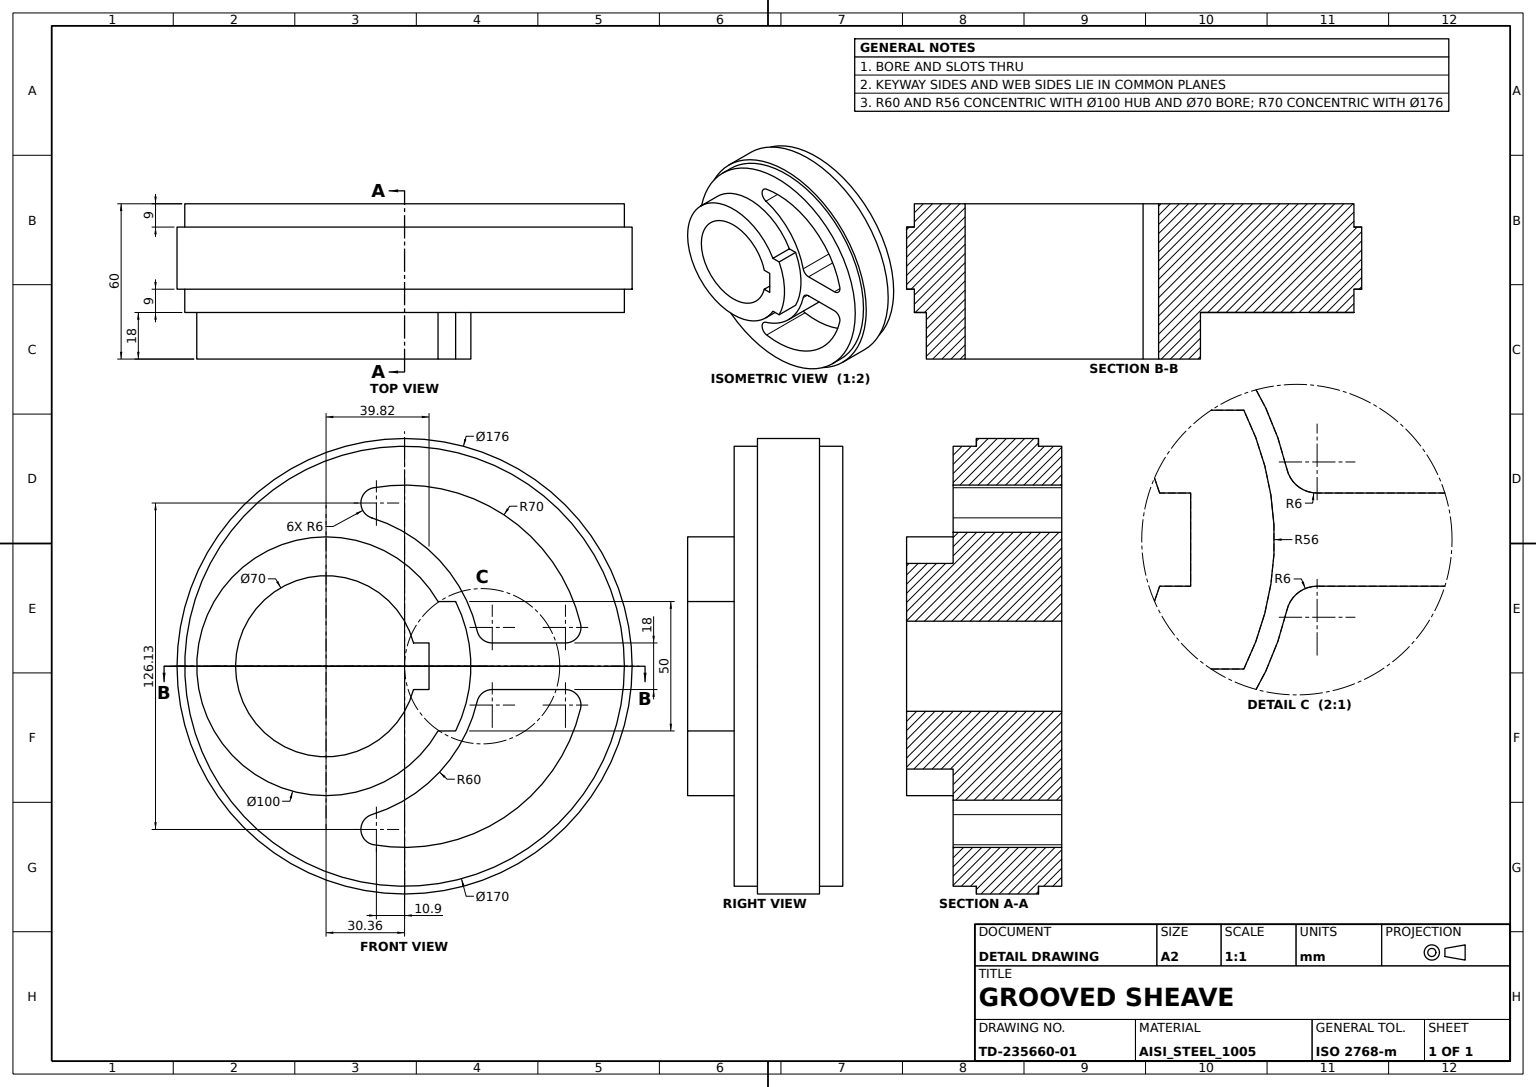
ISO-10303-21;
HEADER;
FILE_DESCRIPTION((''),'2;1');
FILE_NAME('','',(''),(''),'','','');
FILE_SCHEMA(('AUTOMOTIVE_DESIGN'));
ENDSEC;
DATA;
#1=APPLICATION_CONTEXT('');
#2=PRODUCT_CONTEXT('',#1,'mechanical');
#3=PRODUCT('','','',(#2));
#4=PRODUCT_DEFINITION_FORMATION('','',#3);
#5=PRODUCT_DEFINITION_CONTEXT('',#1,'design');
#6=PRODUCT_DEFINITION('','',#4,#5);
#7=PRODUCT_DEFINITION_SHAPE('','',#6);
#8=(LENGTH_UNIT()NAMED_UNIT(*)SI_UNIT(.MILLI.,.METRE.));
#9=(NAMED_UNIT(*)PLANE_ANGLE_UNIT()SI_UNIT($,.RADIAN.));
#10=(NAMED_UNIT(*)SI_UNIT($,.STERADIAN.)SOLID_ANGLE_UNIT());
#11=UNCERTAINTY_MEASURE_WITH_UNIT(LENGTH_MEASURE(0.005),#8,'distance_accuracy_value','');
#12=(GEOMETRIC_REPRESENTATION_CONTEXT(3)GLOBAL_UNCERTAINTY_ASSIGNED_CONTEXT((#11))GLOBAL_UNIT_ASSIGNED_CONTEXT((#8,#9,#10))REPRESENTATION_CONTEXT('',''));
#13=CARTESIAN_POINT('',(0.,85.,12.));
#14=VERTEX_POINT('',#13);
#15=CARTESIAN_POINT('',(0.,0.,12.));
#16=DIRECTION('',(0.,0.,1.));
#17=DIRECTION('',(0.,1.,0.));
#18=AXIS2_PLACEMENT_3D('',#15,#16,#17);
#19=CIRCLE('',#18,85.);
#20=EDGE_CURVE('',#14,#14,#19,.T.);
#21=ORIENTED_EDGE('',*,*,#20,.F.);
#22=EDGE_LOOP('',(#21));
#23=FACE_BOUND('',#22,.T.);
#24=CARTESIAN_POINT('',(0.,88.,12.));
#25=VERTEX_POINT('',#24);
#26=CIRCLE('',#18,88.);
#27=EDGE_CURVE('',#25,#25,#26,.T.);
#28=ORIENTED_EDGE('',*,*,#27,.T.);
#29=EDGE_LOOP('',(#28));
#30=FACE_BOUND('',#29,.T.);
#31=DIRECTION('',(1.,0.,0.));
#32=AXIS2_PLACEMENT_3D('',#15,#16,#31);
#33=PLANE('',#32);
#34=ADVANCED_FACE('',(#23,#30),#33,.T.);
#35=CARTESIAN_POINT('',(-13.636364,28.067483,-21.));
#36=VERTEX_POINT('',#35);
#37=CARTESIAN_POINT('',(-57.331854,-12.668926,-21.));
#38=VERTEX_POINT('',#37);
#39=CARTESIAN_POINT('',(0.,-30.362386,-21.));
#40=AXIS2_PLACEMENT_3D('',#39,#16,#31);
#41=CIRCLE('',#40,60.);
#42=EDGE_CURVE('',#36,#38,#41,.T.);
#43=ORIENTED_EDGE('',*,*,#42,.T.);
#44=CARTESIAN_POINT('',(-57.331854,-12.668926,21.));
#45=VERTEX_POINT('',#44);
#46=CARTESIAN_POINT('',(-57.331854,-12.668926,-54979.));
#47=VECTOR('',#16,1000.);
#48=LINE('',#46,#47);
#49=EDGE_CURVE('',#45,#38,#48,.F.);
#50=ORIENTED_EDGE('',*,*,#49,.F.);
#51=CARTESIAN_POINT('',(-13.636364,28.067483,21.));
#52=VERTEX_POINT('',#51);
#53=CARTESIAN_POINT('',(0.,-30.362386,21.));
#54=DIRECTION('',(0.,0.,-1.));
#55=AXIS2_PLACEMENT_3D('',#53,#54,#31);
#56=CIRCLE('',#55,60.);
#57=EDGE_CURVE('',#45,#52,#56,.T.);
#58=ORIENTED_EDGE('',*,*,#57,.T.);
#59=CARTESIAN_POINT('',(-13.636364,28.067483,-54979.));
#60=LINE('',#59,#47);
#61=EDGE_CURVE('',#52,#36,#60,.F.);
#62=ORIENTED_EDGE('',*,*,#61,.T.);
#63=EDGE_LOOP('',(#43,#50,#58,#62));
#64=FACE_BOUND('',#63,.T.);
#65=CARTESIAN_POINT('',(0.,-30.362386,-54979.));
#66=AXIS2_PLACEMENT_3D('',#65,#16,#31);
#67=CYLINDRICAL_SURFACE('',#66,60.);
#68=ADVANCED_FACE('',(#64),#67,.T.);
#69=CARTESIAN_POINT('',(-9.,3.460683,39.));
#70=VERTEX_POINT('',#69);
#71=CARTESIAN_POINT('',(-9.,3.460683,-21.));
#72=VERTEX_POINT('',#71);
#73=VECTOR('',#54,1000.);
#74=LINE('',#69,#73);
#75=EDGE_CURVE('',#70,#72,#74,.T.);
#76=ORIENTED_EDGE('',*,*,#75,.F.);
#77=CARTESIAN_POINT('',(9.,3.460683,39.));
#78=VERTEX_POINT('',#77);
#79=CARTESIAN_POINT('',(0.,-30.362386,39.));
#80=AXIS2_PLACEMENT_3D('',#79,#54,#31);
#81=CIRCLE('',#80,35.);
#82=EDGE_CURVE('',#78,#70,#81,.T.);
#83=ORIENTED_EDGE('',*,*,#82,.F.);
#84=CARTESIAN_POINT('',(9.,3.460683,-21.));
#85=VERTEX_POINT('',#84);
#86=LINE('',#77,#73);
#87=EDGE_CURVE('',#78,#85,#86,.T.);
#88=ORIENTED_EDGE('',*,*,#87,.T.);
#89=CIRCLE('',#40,35.);
#90=EDGE_CURVE('',#85,#72,#89,.F.);
#91=ORIENTED_EDGE('',*,*,#90,.T.);
#92=EDGE_LOOP('',(#76,#83,#88,#91));
#93=FACE_BOUND('',#92,.T.);
#94=DIRECTION('',(-1.,0.,0.));
#95=AXIS2_PLACEMENT_3D('',#79,#54,#94);
#96=CYLINDRICAL_SURFACE('',#95,35.);
#97=ADVANCED_FACE('',(#93),#96,.F.);
#98=CARTESIAN_POINT('',(68.977387,-11.921415,21.));
#99=VERTEX_POINT('',#98);
#100=CARTESIAN_POINT('',(68.977387,-11.921415,-21.));
#101=VERTEX_POINT('',#100);
#102=CARTESIAN_POINT('',(68.977387,-11.921415,-54979.));
#103=LINE('',#102,#47);
#104=EDGE_CURVE('',#99,#101,#103,.F.);
#105=ORIENTED_EDGE('',*,*,#104,.F.);
#106=CARTESIAN_POINT('',(16.40625,68.050239,21.));
#107=VERTEX_POINT('',#106);
#108=CARTESIAN_POINT('',(0.,0.,21.));
#109=AXIS2_PLACEMENT_3D('',#108,#16,#94);
#110=CIRCLE('',#109,70.);
#111=EDGE_CURVE('',#99,#107,#110,.T.);
#112=ORIENTED_EDGE('',*,*,#111,.T.);
#113=CARTESIAN_POINT('',(16.40625,68.050239,-21.));
#114=VERTEX_POINT('',#113);
#115=CARTESIAN_POINT('',(16.40625,68.050239,-54979.));
#116=LINE('',#115,#47);
#117=EDGE_CURVE('',#107,#114,#116,.F.);
#118=ORIENTED_EDGE('',*,*,#117,.T.);
#119=CARTESIAN_POINT('',(0.,0.,-21.));
#120=AXIS2_PLACEMENT_3D('',#119,#16,#31);
#121=CIRCLE('',#120,70.);
#122=EDGE_CURVE('',#114,#101,#121,.F.);
#123=ORIENTED_EDGE('',*,*,#122,.T.);
#124=EDGE_LOOP('',(#105,#112,#118,#123));
#125=FACE_BOUND('',#124,.T.);
#126=CARTESIAN_POINT('',(0.,0.,-54979.));
#127=AXIS2_PLACEMENT_3D('',#126,#16,#31);
#128=CYLINDRICAL_SURFACE('',#127,70.);
#129=ADVANCED_FACE('',(#125),#128,.F.);
#130=ORIENTED_EDGE('',*,*,#49,.T.);
#131=CARTESIAN_POINT('',(-68.977387,-11.921415,-21.));
#132=VERTEX_POINT('',#131);
#133=CARTESIAN_POINT('',(-63.065039,-10.89958,-21.));
#134=AXIS2_PLACEMENT_3D('',#133,#16,#31);
#135=CIRCLE('',#134,6.);
#136=EDGE_CURVE('',#38,#132,#135,.F.);
#137=ORIENTED_EDGE('',*,*,#136,.T.);
#138=CARTESIAN_POINT('',(-68.977387,-11.921415,21.));
#139=VERTEX_POINT('',#138);
#140=CARTESIAN_POINT('',(-68.977387,-11.921415,-54979.));
#141=LINE('',#140,#47);
#142=EDGE_CURVE('',#139,#132,#141,.F.);
#143=ORIENTED_EDGE('',*,*,#142,.F.);
#144=CARTESIAN_POINT('',(-63.065039,-10.89958,21.));
#145=AXIS2_PLACEMENT_3D('',#144,#16,#31);
#146=CIRCLE('',#145,6.);
#147=EDGE_CURVE('',#139,#45,#146,.T.);
#148=ORIENTED_EDGE('',*,*,#147,.T.);
#149=EDGE_LOOP('',(#130,#137,#143,#148));
#150=FACE_BOUND('',#149,.T.);
#151=CARTESIAN_POINT('',(-63.065039,-10.89958,-54979.));
#152=AXIS2_PLACEMENT_3D('',#151,#16,#31);
#153=CYLINDRICAL_SURFACE('',#152,6.);
#154=ADVANCED_FACE('',(#150),#153,.F.);
#155=CARTESIAN_POINT('',(13.636364,28.067483,21.));
#156=VERTEX_POINT('',#155);
#157=CARTESIAN_POINT('',(57.331854,-12.668926,21.));
#158=VERTEX_POINT('',#157);
#159=AXIS2_PLACEMENT_3D('',#53,#54,#94);
#160=CIRCLE('',#159,60.);
#161=EDGE_CURVE('',#156,#158,#160,.T.);
#162=ORIENTED_EDGE('',*,*,#161,.T.);
#163=CARTESIAN_POINT('',(57.331854,-12.668926,-21.));
#164=VERTEX_POINT('',#163);
#165=CARTESIAN_POINT('',(57.331854,-12.668926,-54979.));
#166=LINE('',#165,#47);
#167=EDGE_CURVE('',#158,#164,#166,.F.);
#168=ORIENTED_EDGE('',*,*,#167,.T.);
#169=CARTESIAN_POINT('',(13.636364,28.067483,-21.));
#170=VERTEX_POINT('',#169);
#171=EDGE_CURVE('',#164,#170,#41,.T.);
#172=ORIENTED_EDGE('',*,*,#171,.T.);
#173=CARTESIAN_POINT('',(13.636364,28.067483,-54979.));
#174=LINE('',#173,#47);
#175=EDGE_CURVE('',#156,#170,#174,.F.);
#176=ORIENTED_EDGE('',*,*,#175,.F.);
#177=EDGE_LOOP('',(#162,#168,#172,#176));
#178=FACE_BOUND('',#177,.T.);
#179=ADVANCED_FACE('',(#178),#67,.T.);
#180=CARTESIAN_POINT('',(-9.,9.460683,39.));
#181=VERTEX_POINT('',#180);
#182=CARTESIAN_POINT('',(9.,9.460683,39.));
#183=VERTEX_POINT('',#182);
#184=VECTOR('',#31,1000.);
#185=LINE('',#180,#184);
#186=EDGE_CURVE('',#181,#183,#185,.T.);
#187=ORIENTED_EDGE('',*,*,#186,.F.);
#188=CARTESIAN_POINT('',(-9.,9.460683,-21.));
#189=VERTEX_POINT('',#188);
#190=LINE('',#180,#73);
#191=EDGE_CURVE('',#181,#189,#190,.T.);
#192=ORIENTED_EDGE('',*,*,#191,.T.);
#193=CARTESIAN_POINT('',(9.,9.460683,-21.));
#194=VERTEX_POINT('',#193);
#195=LINE('',#193,#184);
#196=EDGE_CURVE('',#189,#194,#195,.T.);
#197=ORIENTED_EDGE('',*,*,#196,.T.);
#198=LINE('',#182,#73);
#199=EDGE_CURVE('',#183,#194,#198,.T.);
#200=ORIENTED_EDGE('',*,*,#199,.F.);
#201=EDGE_LOOP('',(#187,#192,#197,#200));
#202=FACE_BOUND('',#201,.T.);
#203=AXIS2_PLACEMENT_3D('',#180,#17,#94);
#204=PLANE('',#203);
#205=ADVANCED_FACE('',(#202),#204,.F.);
#206=CARTESIAN_POINT('',(-9.,62.217361,21.));
#207=VERTEX_POINT('',#206);
#208=CARTESIAN_POINT('',(-9.,62.217361,-21.));
#209=VERTEX_POINT('',#208);
#210=CARTESIAN_POINT('',(-9.,62.217361,-54979.));
#211=LINE('',#210,#47);
#212=EDGE_CURVE('',#207,#209,#211,.F.);
#213=ORIENTED_EDGE('',*,*,#212,.F.);
#214=CARTESIAN_POINT('',(-16.40625,68.050239,21.));
#215=VERTEX_POINT('',#214);
#216=CARTESIAN_POINT('',(-15.,62.217361,21.));
#217=AXIS2_PLACEMENT_3D('',#216,#16,#31);
#218=CIRCLE('',#217,6.);
#219=EDGE_CURVE('',#207,#215,#218,.T.);
#220=ORIENTED_EDGE('',*,*,#219,.T.);
#221=CARTESIAN_POINT('',(-16.40625,68.050239,-21.));
#222=VERTEX_POINT('',#221);
#223=CARTESIAN_POINT('',(-16.40625,68.050239,-54979.));
#224=LINE('',#223,#47);
#225=EDGE_CURVE('',#215,#222,#224,.F.);
#226=ORIENTED_EDGE('',*,*,#225,.T.);
#227=CARTESIAN_POINT('',(-15.,62.217361,-21.));
#228=AXIS2_PLACEMENT_3D('',#227,#16,#31);
#229=CIRCLE('',#228,6.);
#230=EDGE_CURVE('',#222,#209,#229,.F.);
#231=ORIENTED_EDGE('',*,*,#230,.T.);
#232=EDGE_LOOP('',(#213,#220,#226,#231));
#233=FACE_BOUND('',#232,.T.);
#234=CARTESIAN_POINT('',(-15.,62.217361,-54979.));
#235=AXIS2_PLACEMENT_3D('',#234,#16,#31);
#236=CYLINDRICAL_SURFACE('',#235,6.);
#237=ADVANCED_FACE('',(#233),#236,.F.);
#238=CARTESIAN_POINT('',(9.,33.91047,-21.));
#239=VERTEX_POINT('',#238);
#240=CARTESIAN_POINT('',(9.,62.217361,-21.));
#241=VERTEX_POINT('',#240);
#242=VECTOR('',#17,1000.);
#243=LINE('',#240,#242);
#244=EDGE_CURVE('',#239,#241,#243,.T.);
#245=ORIENTED_EDGE('',*,*,#244,.F.);
#246=CARTESIAN_POINT('',(15.,33.91047,-21.));
#247=AXIS2_PLACEMENT_3D('',#246,#16,#31);
#248=CIRCLE('',#247,6.);
#249=EDGE_CURVE('',#170,#239,#248,.F.);
#250=ORIENTED_EDGE('',*,*,#249,.F.);
#251=ORIENTED_EDGE('',*,*,#171,.F.);
#252=CARTESIAN_POINT('',(63.065039,-10.89958,-21.));
#253=AXIS2_PLACEMENT_3D('',#252,#16,#31);
#254=CIRCLE('',#253,6.);
#255=EDGE_CURVE('',#101,#164,#254,.F.);
#256=ORIENTED_EDGE('',*,*,#255,.F.);
#257=ORIENTED_EDGE('',*,*,#122,.F.);
#258=CARTESIAN_POINT('',(15.,62.217361,-21.));
#259=AXIS2_PLACEMENT_3D('',#258,#16,#31);
#260=CIRCLE('',#259,6.);
#261=EDGE_CURVE('',#241,#114,#260,.F.);
#262=ORIENTED_EDGE('',*,*,#261,.F.);
#263=EDGE_LOOP('',(#245,#250,#251,#256,#257,#262));
#264=FACE_BOUND('',#263,.T.);
#265=ORIENTED_EDGE('',*,*,#196,.F.);
#266=LINE('',#188,#242);
#267=EDGE_CURVE('',#72,#189,#266,.T.);
#268=ORIENTED_EDGE('',*,*,#267,.F.);
#269=ORIENTED_EDGE('',*,*,#90,.F.);
#270=DIRECTION('',(0.,-1.,0.));
#271=VECTOR('',#270,1000.);
#272=LINE('',#84,#271);
#273=EDGE_CURVE('',#194,#85,#272,.T.);
#274=ORIENTED_EDGE('',*,*,#273,.F.);
#275=EDGE_LOOP('',(#265,#268,#269,#274));
#276=FACE_BOUND('',#275,.T.);
#277=CARTESIAN_POINT('',(0.,85.,-21.));
#278=VERTEX_POINT('',#277);
#279=AXIS2_PLACEMENT_3D('',#119,#16,#17);
#280=CIRCLE('',#279,85.);
#281=EDGE_CURVE('',#278,#278,#280,.T.);
#282=ORIENTED_EDGE('',*,*,#281,.F.);
#283=EDGE_LOOP('',(#282));
#284=FACE_BOUND('',#283,.T.);
#285=EDGE_CURVE('',#132,#222,#121,.F.);
#286=ORIENTED_EDGE('',*,*,#285,.F.);
#287=ORIENTED_EDGE('',*,*,#136,.F.);
#288=ORIENTED_EDGE('',*,*,#42,.F.);
#289=CARTESIAN_POINT('',(-9.,33.91047,-21.));
#290=VERTEX_POINT('',#289);
#291=CARTESIAN_POINT('',(-15.,33.91047,-21.));
#292=AXIS2_PLACEMENT_3D('',#291,#16,#31);
#293=CIRCLE('',#292,6.);
#294=EDGE_CURVE('',#290,#36,#293,.F.);
#295=ORIENTED_EDGE('',*,*,#294,.F.);
#296=LINE('',#289,#271);
#297=EDGE_CURVE('',#209,#290,#296,.T.);
#298=ORIENTED_EDGE('',*,*,#297,.F.);
#299=ORIENTED_EDGE('',*,*,#230,.F.);
#300=EDGE_LOOP('',(#286,#287,#288,#295,#298,#299));
#301=FACE_BOUND('',#300,.T.);
#302=PLANE('',#120);
#303=ADVANCED_FACE('',(#264,#276,#284,#301),#302,.F.);
#304=CARTESIAN_POINT('',(25.,19.747493,39.));
#305=VERTEX_POINT('',#304);
#306=CARTESIAN_POINT('',(-25.,19.747493,39.));
#307=VERTEX_POINT('',#306);
#308=AXIS2_PLACEMENT_3D('',#79,#16,#31);
#309=CIRCLE('',#308,56.);
#310=EDGE_CURVE('',#305,#307,#309,.T.);
#311=ORIENTED_EDGE('',*,*,#310,.T.);
#312=CARTESIAN_POINT('',(-25.,12.938884,39.));
#313=VERTEX_POINT('',#312);
#314=LINE('',#306,#271);
#315=EDGE_CURVE('',#307,#313,#314,.T.);
#316=ORIENTED_EDGE('',*,*,#315,.T.);
#317=CARTESIAN_POINT('',(25.,12.938884,39.));
#318=VERTEX_POINT('',#317);
#319=CIRCLE('',#308,50.);
#320=EDGE_CURVE('',#313,#318,#319,.T.);
#321=ORIENTED_EDGE('',*,*,#320,.T.);
#322=LINE('',#317,#242);
#323=EDGE_CURVE('',#318,#305,#322,.T.);
#324=ORIENTED_EDGE('',*,*,#323,.T.);
#325=EDGE_LOOP('',(#311,#316,#321,#324));
#326=FACE_BOUND('',#325,.T.);
#327=LINE('',#69,#242);
#328=EDGE_CURVE('',#70,#181,#327,.T.);
#329=ORIENTED_EDGE('',*,*,#328,.T.);
#330=ORIENTED_EDGE('',*,*,#186,.T.);
#331=LINE('',#182,#271);
#332=EDGE_CURVE('',#183,#78,#331,.T.);
#333=ORIENTED_EDGE('',*,*,#332,.T.);
#334=ORIENTED_EDGE('',*,*,#82,.T.);
#335=EDGE_LOOP('',(#329,#330,#333,#334));
#336=FACE_BOUND('',#335,.T.);
#337=PLANE('',#308);
#338=ADVANCED_FACE('',(#326,#336),#337,.T.);
#339=ORIENTED_EDGE('',*,*,#285,.T.);
#340=ORIENTED_EDGE('',*,*,#225,.F.);
#341=AXIS2_PLACEMENT_3D('',#108,#16,#31);
#342=CIRCLE('',#341,70.);
#343=EDGE_CURVE('',#215,#139,#342,.T.);
#344=ORIENTED_EDGE('',*,*,#343,.T.);
#345=ORIENTED_EDGE('',*,*,#142,.T.);
#346=EDGE_LOOP('',(#339,#340,#344,#345));
#347=FACE_BOUND('',#346,.T.);
#348=ADVANCED_FACE('',(#347),#128,.F.);
#349=ORIENTED_EDGE('',*,*,#255,.T.);
#350=ORIENTED_EDGE('',*,*,#167,.F.);
#351=CARTESIAN_POINT('',(63.065039,-10.89958,21.));
#352=AXIS2_PLACEMENT_3D('',#351,#16,#94);
#353=CIRCLE('',#352,6.);
#354=EDGE_CURVE('',#158,#99,#353,.T.);
#355=ORIENTED_EDGE('',*,*,#354,.T.);
#356=ORIENTED_EDGE('',*,*,#104,.T.);
#357=EDGE_LOOP('',(#349,#350,#355,#356));
#358=FACE_BOUND('',#357,.T.);
#359=CARTESIAN_POINT('',(63.065039,-10.89958,-54979.));
#360=AXIS2_PLACEMENT_3D('',#359,#16,#31);
#361=CYLINDRICAL_SURFACE('',#360,6.);
#362=ADVANCED_FACE('',(#358),#361,.F.);
#363=ORIENTED_EDGE('',*,*,#75,.T.);
#364=ORIENTED_EDGE('',*,*,#267,.T.);
#365=ORIENTED_EDGE('',*,*,#191,.F.);
#366=ORIENTED_EDGE('',*,*,#328,.F.);
#367=EDGE_LOOP('',(#363,#364,#365,#366));
#368=FACE_BOUND('',#367,.T.);
#369=AXIS2_PLACEMENT_3D('',#69,#94,#270);
#370=PLANE('',#369);
#371=ADVANCED_FACE('',(#368),#370,.F.);
#372=CARTESIAN_POINT('',(-25.,19.747493,21.));
#373=VERTEX_POINT('',#372);
#374=LINE('',#306,#73);
#375=EDGE_CURVE('',#307,#373,#374,.T.);
#376=ORIENTED_EDGE('',*,*,#375,.F.);
#377=ORIENTED_EDGE('',*,*,#310,.F.);
#378=CARTESIAN_POINT('',(25.,19.747493,21.));
#379=VERTEX_POINT('',#378);
#380=LINE('',#304,#73);
#381=EDGE_CURVE('',#305,#379,#380,.T.);
#382=ORIENTED_EDGE('',*,*,#381,.T.);
#383=AXIS2_PLACEMENT_3D('',#53,#16,#31);
#384=CIRCLE('',#383,56.);
#385=EDGE_CURVE('',#379,#373,#384,.T.);
#386=ORIENTED_EDGE('',*,*,#385,.T.);
#387=EDGE_LOOP('',(#376,#377,#382,#386));
#388=FACE_BOUND('',#387,.T.);
#389=CYLINDRICAL_SURFACE('',#95,56.);
#390=ADVANCED_FACE('',(#388),#389,.T.);
#391=ORIENTED_EDGE('',*,*,#27,.F.);
#392=EDGE_LOOP('',(#391));
#393=FACE_BOUND('',#392,.T.);
#394=CARTESIAN_POINT('',(0.,88.,-12.));
#395=VERTEX_POINT('',#394);
#396=CARTESIAN_POINT('',(0.,0.,-12.));
#397=AXIS2_PLACEMENT_3D('',#396,#16,#17);
#398=CIRCLE('',#397,88.);
#399=EDGE_CURVE('',#395,#395,#398,.T.);
#400=ORIENTED_EDGE('',*,*,#399,.T.);
#401=EDGE_LOOP('',(#400));
#402=FACE_BOUND('',#401,.T.);
#403=AXIS2_PLACEMENT_3D('',#15,#54,#94);
#404=CYLINDRICAL_SURFACE('',#403,88.);
#405=ADVANCED_FACE('',(#393,#402),#404,.T.);
#406=ORIENTED_EDGE('',*,*,#249,.T.);
#407=CARTESIAN_POINT('',(9.,33.91047,21.));
#408=VERTEX_POINT('',#407);
#409=CARTESIAN_POINT('',(9.,33.91047,-54979.));
#410=LINE('',#409,#47);
#411=EDGE_CURVE('',#408,#239,#410,.F.);
#412=ORIENTED_EDGE('',*,*,#411,.F.);
#413=CARTESIAN_POINT('',(15.,33.91047,21.));
#414=AXIS2_PLACEMENT_3D('',#413,#16,#94);
#415=CIRCLE('',#414,6.);
#416=EDGE_CURVE('',#408,#156,#415,.T.);
#417=ORIENTED_EDGE('',*,*,#416,.T.);
#418=ORIENTED_EDGE('',*,*,#175,.T.);
#419=EDGE_LOOP('',(#406,#412,#417,#418));
#420=FACE_BOUND('',#419,.T.);
#421=CARTESIAN_POINT('',(15.,33.91047,-54979.));
#422=AXIS2_PLACEMENT_3D('',#421,#16,#31);
#423=CYLINDRICAL_SURFACE('',#422,6.);
#424=ADVANCED_FACE('',(#420),#423,.F.);
#425=CARTESIAN_POINT('',(0.,85.,21.));
#426=VERTEX_POINT('',#425);
#427=AXIS2_PLACEMENT_3D('',#108,#16,#17);
#428=CIRCLE('',#427,85.);
#429=EDGE_CURVE('',#426,#426,#428,.T.);
#430=ORIENTED_EDGE('',*,*,#429,.T.);
#431=EDGE_LOOP('',(#430));
#432=FACE_BOUND('',#431,.T.);
#433=ORIENTED_EDGE('',*,*,#416,.F.);
#434=CARTESIAN_POINT('',(9.,62.217361,21.));
#435=VERTEX_POINT('',#434);
#436=LINE('',#434,#271);
#437=EDGE_CURVE('',#435,#408,#436,.T.);
#438=ORIENTED_EDGE('',*,*,#437,.F.);
#439=CARTESIAN_POINT('',(15.,62.217361,21.));
#440=AXIS2_PLACEMENT_3D('',#439,#16,#94);
#441=CIRCLE('',#440,6.);
#442=EDGE_CURVE('',#107,#435,#441,.T.);
#443=ORIENTED_EDGE('',*,*,#442,.F.);
#444=ORIENTED_EDGE('',*,*,#111,.F.);
#445=ORIENTED_EDGE('',*,*,#354,.F.);
#446=ORIENTED_EDGE('',*,*,#161,.F.);
#447=EDGE_LOOP('',(#433,#438,#443,#444,#445,#446));
#448=FACE_BOUND('',#447,.T.);
#449=ORIENTED_EDGE('',*,*,#57,.F.);
#450=ORIENTED_EDGE('',*,*,#147,.F.);
#451=ORIENTED_EDGE('',*,*,#343,.F.);
#452=ORIENTED_EDGE('',*,*,#219,.F.);
#453=CARTESIAN_POINT('',(-9.,33.91047,21.));
#454=VERTEX_POINT('',#453);
#455=LINE('',#453,#242);
#456=EDGE_CURVE('',#454,#207,#455,.T.);
#457=ORIENTED_EDGE('',*,*,#456,.F.);
#458=CARTESIAN_POINT('',(-15.,33.91047,21.));
#459=AXIS2_PLACEMENT_3D('',#458,#16,#31);
#460=CIRCLE('',#459,6.);
#461=EDGE_CURVE('',#52,#454,#460,.T.);
#462=ORIENTED_EDGE('',*,*,#461,.F.);
#463=EDGE_LOOP('',(#449,#450,#451,#452,#457,#462));
#464=FACE_BOUND('',#463,.T.);
#465=CARTESIAN_POINT('',(25.,12.938884,21.));
#466=VERTEX_POINT('',#465);
#467=LINE('',#465,#242);
#468=EDGE_CURVE('',#466,#379,#467,.T.);
#469=ORIENTED_EDGE('',*,*,#468,.F.);
#470=CARTESIAN_POINT('',(-25.,12.938884,21.));
#471=VERTEX_POINT('',#470);
#472=CIRCLE('',#383,50.);
#473=EDGE_CURVE('',#471,#466,#472,.T.);
#474=ORIENTED_EDGE('',*,*,#473,.F.);
#475=LINE('',#372,#271);
#476=EDGE_CURVE('',#373,#471,#475,.T.);
#477=ORIENTED_EDGE('',*,*,#476,.F.);
#478=ORIENTED_EDGE('',*,*,#385,.F.);
#479=EDGE_LOOP('',(#469,#474,#477,#478));
#480=FACE_BOUND('',#479,.T.);
#481=PLANE('',#341);
#482=ADVANCED_FACE('',(#432,#448,#464,#480),#481,.T.);
#483=ORIENTED_EDGE('',*,*,#476,.T.);
#484=LINE('',#312,#73);
#485=EDGE_CURVE('',#313,#471,#484,.T.);
#486=ORIENTED_EDGE('',*,*,#485,.F.);
#487=ORIENTED_EDGE('',*,*,#315,.F.);
#488=ORIENTED_EDGE('',*,*,#375,.T.);
#489=EDGE_LOOP('',(#483,#486,#487,#488));
#490=FACE_BOUND('',#489,.T.);
#491=AXIS2_PLACEMENT_3D('',#306,#31,#54);
#492=PLANE('',#491);
#493=ADVANCED_FACE('',(#490),#492,.F.);
#494=ORIENTED_EDGE('',*,*,#461,.T.);
#495=CARTESIAN_POINT('',(-9.,33.91047,-54979.));
#496=LINE('',#495,#47);
#497=EDGE_CURVE('',#454,#290,#496,.F.);
#498=ORIENTED_EDGE('',*,*,#497,.T.);
#499=ORIENTED_EDGE('',*,*,#294,.T.);
#500=ORIENTED_EDGE('',*,*,#61,.F.);
#501=EDGE_LOOP('',(#494,#498,#499,#500));
#502=FACE_BOUND('',#501,.T.);
#503=CARTESIAN_POINT('',(-15.,33.91047,-54979.));
#504=AXIS2_PLACEMENT_3D('',#503,#16,#31);
#505=CYLINDRICAL_SURFACE('',#504,6.);
#506=ADVANCED_FACE('',(#502),#505,.F.);
#507=ORIENTED_EDGE('',*,*,#429,.F.);
#508=EDGE_LOOP('',(#507));
#509=FACE_BOUND('',#508,.T.);
#510=ORIENTED_EDGE('',*,*,#20,.T.);
#511=EDGE_LOOP('',(#510));
#512=FACE_BOUND('',#511,.T.);
#513=AXIS2_PLACEMENT_3D('',#108,#54,#94);
#514=CYLINDRICAL_SURFACE('',#513,85.);
#515=ADVANCED_FACE('',(#509,#512),#514,.T.);
#516=ORIENTED_EDGE('',*,*,#468,.T.);
#517=ORIENTED_EDGE('',*,*,#381,.F.);
#518=ORIENTED_EDGE('',*,*,#323,.F.);
#519=LINE('',#317,#73);
#520=EDGE_CURVE('',#318,#466,#519,.T.);
#521=ORIENTED_EDGE('',*,*,#520,.T.);
#522=EDGE_LOOP('',(#516,#517,#518,#521));
#523=FACE_BOUND('',#522,.T.);
#524=AXIS2_PLACEMENT_3D('',#317,#94,#270);
#525=PLANE('',#524);
#526=ADVANCED_FACE('',(#523),#525,.F.);
#527=ORIENTED_EDGE('',*,*,#485,.T.);
#528=ORIENTED_EDGE('',*,*,#473,.T.);
#529=ORIENTED_EDGE('',*,*,#520,.F.);
#530=ORIENTED_EDGE('',*,*,#320,.F.);
#531=EDGE_LOOP('',(#527,#528,#529,#530));
#532=FACE_BOUND('',#531,.T.);
#533=CYLINDRICAL_SURFACE('',#95,50.);
#534=ADVANCED_FACE('',(#532),#533,.T.);
#535=CARTESIAN_POINT('',(85.,0.,-12.));
#536=VERTEX_POINT('',#535);
#537=AXIS2_PLACEMENT_3D('',#396,#16,#31);
#538=CIRCLE('',#537,85.);
#539=EDGE_CURVE('',#536,#536,#538,.T.);
#540=ORIENTED_EDGE('',*,*,#539,.F.);
#541=EDGE_LOOP('',(#540));
#542=FACE_BOUND('',#541,.T.);
#543=ORIENTED_EDGE('',*,*,#281,.T.);
#544=EDGE_LOOP('',(#543));
#545=FACE_BOUND('',#544,.T.);
#546=ADVANCED_FACE('',(#542,#545),#514,.T.);
#547=ORIENTED_EDGE('',*,*,#437,.T.);
#548=ORIENTED_EDGE('',*,*,#411,.T.);
#549=ORIENTED_EDGE('',*,*,#244,.T.);
#550=CARTESIAN_POINT('',(9.,62.217361,-54979.));
#551=LINE('',#550,#47);
#552=EDGE_CURVE('',#435,#241,#551,.F.);
#553=ORIENTED_EDGE('',*,*,#552,.F.);
#554=EDGE_LOOP('',(#547,#548,#549,#553));
#555=FACE_BOUND('',#554,.T.);
#556=AXIS2_PLACEMENT_3D('',#550,#94,#16);
#557=PLANE('',#556);
#558=ADVANCED_FACE('',(#555),#557,.F.);
#559=ORIENTED_EDGE('',*,*,#399,.F.);
#560=EDGE_LOOP('',(#559));
#561=FACE_BOUND('',#560,.T.);
#562=ORIENTED_EDGE('',*,*,#539,.T.);
#563=EDGE_LOOP('',(#562));
#564=FACE_BOUND('',#563,.T.);
#565=PLANE('',#537);
#566=ADVANCED_FACE('',(#561,#564),#565,.F.);
#567=ORIENTED_EDGE('',*,*,#552,.T.);
#568=ORIENTED_EDGE('',*,*,#261,.T.);
#569=ORIENTED_EDGE('',*,*,#117,.F.);
#570=ORIENTED_EDGE('',*,*,#442,.T.);
#571=EDGE_LOOP('',(#567,#568,#569,#570));
#572=FACE_BOUND('',#571,.T.);
#573=CARTESIAN_POINT('',(15.,62.217361,-54979.));
#574=AXIS2_PLACEMENT_3D('',#573,#16,#31);
#575=CYLINDRICAL_SURFACE('',#574,6.);
#576=ADVANCED_FACE('',(#572),#575,.F.);
#577=ORIENTED_EDGE('',*,*,#199,.T.);
#578=ORIENTED_EDGE('',*,*,#273,.T.);
#579=ORIENTED_EDGE('',*,*,#87,.F.);
#580=ORIENTED_EDGE('',*,*,#332,.F.);
#581=EDGE_LOOP('',(#577,#578,#579,#580));
#582=FACE_BOUND('',#581,.T.);
#583=AXIS2_PLACEMENT_3D('',#182,#31,#17);
#584=PLANE('',#583);
#585=ADVANCED_FACE('',(#582),#584,.F.);
#586=ORIENTED_EDGE('',*,*,#456,.T.);
#587=ORIENTED_EDGE('',*,*,#212,.T.);
#588=ORIENTED_EDGE('',*,*,#297,.T.);
#589=ORIENTED_EDGE('',*,*,#497,.F.);
#590=EDGE_LOOP('',(#586,#587,#588,#589));
#591=FACE_BOUND('',#590,.T.);
#592=AXIS2_PLACEMENT_3D('',#495,#31,#17);
#593=PLANE('',#592);
#594=ADVANCED_FACE('',(#591),#593,.F.);
#595=CLOSED_SHELL('',(#34,#68,#97,#129,#154,#179,#205,#237,#303,#338,#348,#362,#371,#390,#405,#424,#482,#493,#506,#515,#526,#534,#546,#558,#566,#576,#585,#594));
#596=MANIFOLD_SOLID_BREP('',#595);
#597=ADVANCED_BREP_SHAPE_REPRESENTATION('',(#596),#12);
#598=SHAPE_DEFINITION_REPRESENTATION(#7,#597);
ENDSEC;
END-ISO-10303-21;
